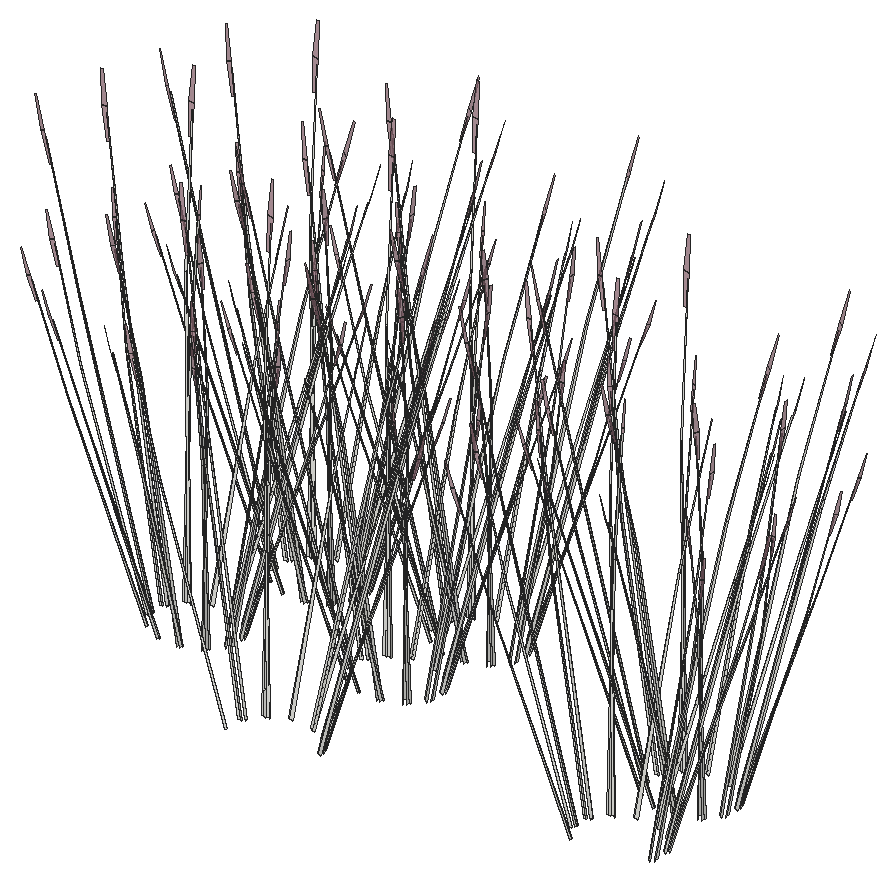
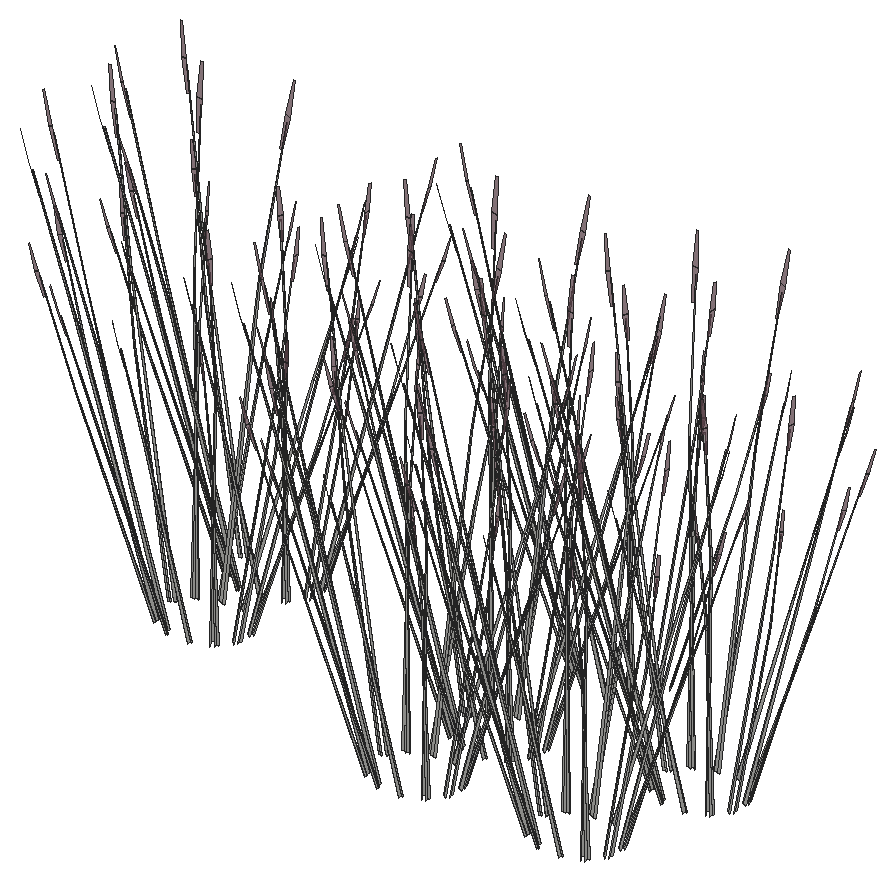
# SketchUp Ruby script. Lengths in inches.
U = 1.inch
M = Sketchup.active_model
def pt(a) = Geom::Point3d.new(a.map { |v| v * U })
def face(e, loops, mat)
  f = e.add_face(loops[0].map { |a| pt(a) })
  loops[1..].each { |l| e.add_face(l.map { |a| pt(a) }).erase! }
  f.material = f.back_material = mat if mat
  f
end
# faces: each face lists its corners as indices into pts; further lists are holes
def faces(e, pts, list, mat = nil) = list.each { |f| face(e, (f[0].is_a?(Array) ? f : [f]).map { |l| l.map { |i| pts[i] } }, mat) }
# xy, xz, yz: faces in a plane at the given z, y or x. An outline is a flat list of corners, or four numbers for a rectangle; further outlines are holes
def ring(l) = l.size == 4 ? [[l[0], l[1]], [l[2], l[1]], [l[2], l[3]], [l[0], l[3]]] : l.each_slice(2).to_a
def flat(e, list, mat, &to3) = list.each { |f| face(e, (f[0].is_a?(Array) ? f : [f]).map { |l| ring(l).map { |u, v| to3.(u, v) } }, mat) }
def xy(e, z, list, mat = nil) = flat(e, list, mat) { |x, y| [x, y, z] }
def xz(e, y, list, mat = nil) = flat(e, list, mat) { |x, z| [x, y, z] }
def yz(e, x, list, mat = nil) = flat(e, list, mat) { |y, z| [x, y, z] }
def lines(e, pts, list) = list.each { |a, b| e.add_line(pt(pts[a]), pt(pts[b])) }
# prism: a flat outline (further loops are holes) pulled along v
def prism(e, loops, v, mat = nil)
  f = face(e, loops, mat); d = Geom::Vector3d.new(v.map { |x| x * U })
  f.pushpull(f.normal.samedirection?(d) ? d.length : -d.length)
end
def box(e, o, s, mat = nil) = prism(e, [[o, [o[0] + s[0], o[1], o[2]], [o[0] + s[0], o[1] + s[1], o[2]], [o[0], o[1] + s[1], o[2]]]], [0, 0, s[2]], mat)
def at(x, y, z, deg = 0) = Geom::Transformation.translation(pt([x, y, z])) * Geom::Transformation.rotation(ORIGIN, Z_AXIS, deg.degrees)
def axes(o, x, y, z) = Geom::Transformation.new([*x, 0, *y, 0, *z, 0, *pt(o).to_a, 1])
def part(name) = M.definitions.add(name)
# library, detail: a bought-in or finely detailed component or shape, given as its bounding box
def library(name, o, s) = part(name).tap { |d| box(d.entities, o, s) }
def detail(e, o, s) = box(e.add_group.entities, o, s)
def put(e, d, t, mat = nil) = e.add_instance(d, t).tap { |i| i.material = mat if mat }
def group(e, t, mat = nil) = e.add_group.tap { |g| g.transformation = t; g.material = mat if mat }.entities
root = M.entities
M.materials.add("LightPink_Translucent").color = [144, 107, 117]
M.materials["LightPink_Translucent"].alpha = 0.75
c1 = part("blade")
p = [[2.15,0.21,22],[0,0.17,0],[0.09,0.45,0],[2.18,0.31,22],[2.29,0.31,22],[0.38,0.45,0],
  [2.48,0.24,33],[2.49,0.24,33],[2.48,0.22,33]]
faces(c1.entities,p,[[0,1,2,3],[4,5,2,3],[6,3,4,7],[8,0,3,6]])
c2 = part("seeds")
p = [[0.3,-0.1,1.38],[-0.01,-0.03,1.59],[-0.01,-0.03,0.03],[0.14,-0.07,-0.07],[0.29,-0.03,3],[0.15,0.01,3.11]]
faces(c2.entities,p,[[0,1,2,3],[1,0,4,5]],"LightPink_Translucent")
c3 = part("blade with seeds")
put(c3.entities,c1,at(0,0,0))
put(c3.entities,c2,axes([2.4,0.25,30.99],[1.5799,-0.05474,1.17369],[-0.12525,1.92788,0.29478],[-0.07173,-0.02425,1.56792]))
put(root,c3,axes([674.05,332.48,513.93],[-0.23895,-0.38931,0.05337],[0.43573,-0.19055,0.42015],[-0.19208,0.0376,0.64067]))
put(root,c3,axes([696.97,334.57,513.93],[0.03276,-0.43418,0.05337],[0.49468,0.0119,0.42015],[-0.18949,-0.04543,0.64067]))
put(root,c3,axes([680.24,333.61,513.93],[0.23895,0.38931,0.05337],[-0.43573,0.19055,0.42015],[0.19208,-0.0376,0.64067]))
put(root,c3,axes([680.2,333.47,513.93],[-0.18381,0.5206,0.39842],[-0.60429,-0.17802,0.32852],[0.23764,-0.03129,0.82444]))
put(root,c3,axes([702.34,335.55,513.93],[0.44663,0.24013,0.05337],[-0.26003,0.34195,0.42015],[0.14319,-0.11055,0.64067]))
put(root,c3,axes([702.21,335.45,513.93],[0.16135,0.52549,0.39842],[-0.63294,0.0912,0.32852],[0.18654,-0.12359,0.82444]))
put(root,c3,axes([666.05,338.03,513.93],[0.64106,0.14927,0.39842],[-0.21921,0.49074,0.32852],[-0.03852,-0.19299,0.82444]))
put(root,c3,axes([666.22,337.99,513.93],[0.47939,-0.19405,0.05337],[0.23464,0.35385,0.42015],[-0.0463,-0.15598,0.64067]))
put(root,c3,axes([674.24,333.91,513.93],[-0.16135,-0.52549,0.39842],[0.63294,-0.0912,0.32852],[-0.18654,0.12359,0.82444]))
put(root,c3,axes([674.11,333.81,513.93],[-0.44663,-0.24013,0.05337],[0.26003,-0.34195,0.42015],[-0.14319,0.11055,0.64067]))
put(root,c3,axes([664.57,338.04,513.93],[0.29569,-0.36271,0.05337],[0.42107,0.21117,0.42015],[-0.13613,-0.11629,0.64067]))
put(root,c3,axes([696.25,335.89,513.93],[0.18381,-0.5206,0.39842],[0.60429,0.17802,0.32852],[-0.23764,0.03129,0.82444]))
put(root,c3,axes([696.21,335.75,513.93],[-0.23895,-0.38931,0.05337],[0.43573,-0.19055,0.42015],[-0.19208,0.0376,0.64067]))
put(root,c3,axes([667.5,338.57,513.93],[0.46327,0.38957,0.39842],[-0.49199,0.33598,0.32852],[0.08546,-0.18277,0.82444]))
put(root,c3,axes([667.67,338.61,513.93],[0.53464,0.0266,0.05337],[-0.01466,0.40172,0.42015],[0.05594,-0.15388,0.64067]))
put(root,c3,axes([679.48,334.79,513.93],[-0.03276,0.43418,0.05337],[-0.49468,-0.0119,0.42015],[0.18949,0.04543,0.64067]))
put(root,c3,axes([679.53,334.65,513.93],[-0.47971,0.37622,0.39842],[-0.41372,-0.39954,0.32852],[0.22506,0.0694,0.82444]))
put(root,c3,axes([702.41,336.88,513.93],[0.23895,0.38931,0.05337],[-0.43573,0.19055,0.42015],[0.19208,-0.0376,0.64067]))
put(root,c3,axes([702.36,336.75,513.93],[-0.18381,0.5206,0.39842],[-0.60429,-0.17802,0.32852],[0.23764,-0.03129,0.82444]))
put(root,c3,axes([678.66,340.24,513.93],[0.64106,0.14927,0.39842],[-0.21921,0.49074,0.32852],[-0.03852,-0.19299,0.82444]))
put(root,c3,axes([699.83,340.24,513.93],[0.64106,0.14927,0.39842],[-0.21921,0.49074,0.32852],[-0.03852,-0.19299,0.82444]))
put(root,c3,axes([678.83,340.2,513.93],[0.47939,-0.19405,0.05337],[0.23464,0.35385,0.42015],[-0.0463,-0.15598,0.64067]))
put(root,c3,axes([700,340.2,513.93],[0.47939,-0.19405,0.05337],[0.23464,0.35385,0.42015],[-0.0463,-0.15598,0.64067]))
put(root,c3,axes([663.19,338.76,513.93],[0.03276,-0.43418,0.05337],[0.49468,0.0119,0.42015],[-0.18949,-0.04543,0.64067]))
put(root,c3,axes([674.99,334.9375,513.93],[-0.53464,-0.0266,0.05337],[0.01466,-0.40172,0.42015],[-0.05594,0.15388,0.64067]))
put(root,c3,axes([675.16,334.97,513.93],[-0.46327,-0.38957,0.39842],[0.49199,-0.33598,0.32852],[-0.08546,0.18277,0.82444]))
put(root,c3,axes([677.1875,340.26,513.93],[0.29569,-0.36271,0.05337],[0.42107,0.21117,0.42015],[-0.13613,-0.11629,0.64067]))
put(root,c3,axes([698.36,340.26,513.93],[0.29569,-0.36271,0.05337],[0.42107,0.21117,0.42015],[-0.13613,-0.11629,0.64067]))
put(root,c3,axes([678.09,335.5,513.93],[-0.29569,0.36271,0.05337],[-0.42107,-0.21117,0.42015],[0.13613,0.11629,0.64067]))
put(root,c3,axes([680.12,340.79,513.93],[0.46327,0.38957,0.39842],[-0.49199,0.33598,0.32852],[0.08546,-0.18277,0.82444]))
put(root,c3,axes([701.29,340.79,513.93],[0.46327,0.38957,0.39842],[-0.49199,0.33598,0.32852],[0.08546,-0.18277,0.82444]))
put(root,c3,axes([668.55,339.74,513.93],[0.44663,0.24013,0.05337],[-0.26003,0.34195,0.42015],[0.14319,-0.11055,0.64067]))
put(root,c3,axes([680.29,340.82,513.93],[0.53464,0.0266,0.05337],[-0.01466,0.40172,0.42015],[0.05594,-0.15388,0.64067]))
put(root,c3,axes([701.46,340.82,513.93],[0.53464,0.0266,0.05337],[-0.01466,0.40172,0.42015],[0.05594,-0.15388,0.64067]))
put(root,c3,axes([668.43,339.64,513.93],[0.16135,0.52549,0.39842],[-0.63294,0.0912,0.32852],[0.18654,-0.12359,0.82444]))
put(root,c3,axes([678.22,335.4,513.93],[-0.64708,0.13103,0.39842],[-0.1123,-0.514,0.32852],[0.15218,0.15149,0.82444]))
put(root,c3,axes([676.45,335.56,513.93],[-0.47939,0.19405,0.05337],[-0.23464,-0.35385,0.42015],[0.0463,0.15598,0.64067]))
put(root,c3,axes([696.4,337.1875,513.93],[-0.16135,-0.52549,0.39842],[0.63294,-0.0912,0.32852],[-0.18654,0.12359,0.82444]))
put(root,c3,axes([696.28,337.09,513.93],[-0.44663,-0.24013,0.05337],[0.26003,-0.34195,0.42015],[-0.14319,0.11055,0.64067]))
put(root,c3,axes([701.64,338.07,513.93],[-0.03276,0.43418,0.05337],[-0.49468,-0.0119,0.42015],[0.18949,0.04543,0.64067]))
put(root,c3,axes([675.8,340.97,513.93],[0.03276,-0.43418,0.05337],[0.49468,0.0119,0.42015],[-0.18949,-0.04543,0.64067]))
put(root,c3,axes([696.97,340.97,513.93],[0.03276,-0.43418,0.05337],[0.49468,0.0119,0.42015],[-0.18949,-0.04543,0.64067]))
put(root,c3,axes([701.6875,337.93,513.93],[-0.47971,0.37622,0.39842],[-0.41372,-0.39954,0.32852],[0.22506,0.0694,0.82444]))
put(root,c3,axes([662.47,340.08,513.93],[0.18381,-0.5206,0.39842],[0.60429,0.17802,0.32852],[-0.23764,0.03129,0.82444]))
put(root,c3,axes([662.42,339.94,513.93],[-0.23895,-0.38931,0.05337],[0.43573,-0.19055,0.42015],[-0.19208,0.0376,0.64067]))
put(root,c3,axes([681.17,341.95,513.93],[0.44663,0.24013,0.05337],[-0.26003,0.34195,0.42015],[0.14319,-0.11055,0.64067]))
put(root,c3,axes([702.34,341.95,513.93],[0.44663,0.24013,0.05337],[-0.26003,0.34195,0.42015],[0.14319,-0.11055,0.64067]))
put(root,c3,axes([681.04,341.85,513.93],[0.16135,0.52549,0.39842],[-0.63294,0.0912,0.32852],[0.18654,-0.12359,0.82444]))
put(root,c3,axes([702.21,341.85,513.93],[0.16135,0.52549,0.39842],[-0.63294,0.0912,0.32852],[0.18654,-0.12359,0.82444]))
put(root,c3,axes([697.15,338.21,513.93],[-0.53464,-0.0266,0.05337],[0.01466,-0.40172,0.42015],[-0.05594,0.15388,0.64067]))
put(root,c3,axes([697.32,338.25,513.93],[-0.46327,-0.38957,0.39842],[0.49199,-0.33598,0.32852],[-0.08546,0.18277,0.82444]))
put(root,c3,axes([668.62,341.07,513.93],[0.23895,0.38931,0.05337],[-0.43573,0.19055,0.42015],[0.19208,-0.0376,0.64067]))
put(root,c3,axes([668.57,340.93,513.93],[-0.18381,0.5206,0.39842],[-0.60429,-0.17802,0.32852],[0.23764,-0.03129,0.82444]))
put(root,c3,axes([700.25,338.78,513.93],[-0.29569,0.36271,0.05337],[-0.42107,-0.21117,0.42015],[0.13613,0.11629,0.64067]))
put(root,c3,axes([700.375,338.68,513.93],[-0.64708,0.13103,0.39842],[-0.1123,-0.514,0.32852],[0.15218,0.15149,0.82444]))
put(root,c3,axes([698.61,338.83,513.93],[-0.47939,0.19405,0.05337],[-0.23464,-0.35385,0.42015],[0.0463,0.15598,0.64067]))
put(root,c3,axes([675.08,342.29,513.93],[0.18381,-0.5206,0.39842],[0.60429,0.17802,0.32852],[-0.23764,0.03129,0.82444]))
put(root,c3,axes([696.25,342.29,513.93],[0.18381,-0.5206,0.39842],[0.60429,0.17802,0.32852],[-0.23764,0.03129,0.82444]))
put(root,c3,axes([675.04,342.15,513.93],[-0.23895,-0.38931,0.05337],[0.43573,-0.19055,0.42015],[-0.19208,0.0376,0.64067]))
put(root,c3,axes([696.21,342.15,513.93],[-0.23895,-0.38931,0.05337],[0.43573,-0.19055,0.42015],[-0.19208,0.0376,0.64067]))
put(root,c3,axes([662.61,341.375,513.93],[-0.16135,-0.52549,0.39842],[0.63294,-0.0912,0.32852],[-0.18654,0.12359,0.82444]))
put(root,c3,axes([662.49,341.27,513.93],[-0.44663,-0.24013,0.05337],[0.26003,-0.34195,0.42015],[-0.14319,0.11055,0.64067]))
put(root,c3,axes([668.3,346.37,513.93],[0.64106,0.14927,0.39842],[-0.21921,0.49074,0.32852],[-0.03852,-0.19299,0.82444]))
put(root,c3,axes([681.23,343.28,513.93],[0.23895,0.38931,0.05337],[-0.43573,0.19055,0.42015],[0.19208,-0.0376,0.64067]))
put(root,c3,axes([702.41,343.28,513.93],[0.23895,0.38931,0.05337],[-0.43573,0.19055,0.42015],[0.19208,-0.0376,0.64067]))
put(root,c3,axes([681.1875,343.15,513.93],[-0.18381,0.5206,0.39842],[-0.60429,-0.17802,0.32852],[0.23764,-0.03129,0.82444]))
put(root,c3,axes([702.36,343.15,513.93],[-0.18381,0.5206,0.39842],[-0.60429,-0.17802,0.32852],[0.23764,-0.03129,0.82444]))
put(root,c3,axes([668.47,346.33,513.93],[0.47939,-0.19405,0.05337],[0.23464,0.35385,0.42015],[-0.0463,-0.15598,0.64067]))
put(root,c3,axes([679.61,346.57,513.93],[0.64106,0.14927,0.39842],[-0.21921,0.49074,0.32852],[-0.03852,-0.19299,0.82444]))
put(root,c3,axes([679.78,346.53,513.93],[0.47939,-0.19405,0.05337],[0.23464,0.35385,0.42015],[-0.0463,-0.15598,0.64067]))
put(root,c3,axes([667.85,342.25,513.93],[-0.03276,0.43418,0.05337],[-0.49468,-0.0119,0.42015],[0.18949,0.04543,0.64067]))
put(root,c3,axes([666.83,346.39,513.93],[0.29569,-0.36271,0.05337],[0.42107,0.21117,0.42015],[-0.13613,-0.11629,0.64067]))
put(root,c3,axes([667.9,342.12,513.93],[-0.47971,0.37622,0.39842],[-0.41372,-0.39954,0.32852],[0.22506,0.0694,0.82444]))
put(root,c3,axes([678.14,346.59,513.93],[0.29569,-0.36271,0.05337],[0.42107,0.21117,0.42015],[-0.13613,-0.11629,0.64067]))
put(root,c3,axes([669.76,346.91,513.93],[0.46327,0.38957,0.39842],[-0.49199,0.33598,0.32852],[0.08546,-0.18277,0.82444]))
put(root,c3,axes([669.93,346.95,513.93],[0.53464,0.0266,0.05337],[-0.01466,0.40172,0.42015],[0.05594,-0.15388,0.64067]))
put(root,c3,axes([681.07,347.12,513.93],[0.46327,0.38957,0.39842],[-0.49199,0.33598,0.32852],[0.08546,-0.18277,0.82444]))
put(root,c3,axes([681.24,347.15,513.93],[0.53464,0.0266,0.05337],[-0.01466,0.40172,0.42015],[0.05594,-0.15388,0.64067]))
put(root,c3,axes([675.23,343.59,513.93],[-0.16135,-0.52549,0.39842],[0.63294,-0.0912,0.32852],[-0.18654,0.12359,0.82444]))
put(root,c3,axes([696.4,343.59,513.93],[-0.16135,-0.52549,0.39842],[0.63294,-0.0912,0.32852],[-0.18654,0.12359,0.82444]))
put(root,c3,axes([663.37,342.4,513.93],[-0.53464,-0.0266,0.05337],[0.01466,-0.40172,0.42015],[-0.05594,0.15388,0.64067]))
put(root,c3,axes([675.1,343.49,513.93],[-0.44663,-0.24013,0.05337],[0.26003,-0.34195,0.42015],[-0.14319,0.11055,0.64067]))
put(root,c3,axes([696.28,343.49,513.93],[-0.44663,-0.24013,0.05337],[0.26003,-0.34195,0.42015],[-0.14319,0.11055,0.64067]))
put(root,c3,axes([663.54,342.4375,513.93],[-0.46327,-0.38957,0.39842],[0.49199,-0.33598,0.32852],[-0.08546,0.18277,0.82444]))
put(root,c3,axes([666.47,342.97,513.93],[-0.29569,0.36271,0.05337],[-0.42107,-0.21117,0.42015],[0.13613,0.11629,0.64067]))
put(root,c3,axes([665.44,347.1,513.93],[0.03276,-0.43418,0.05337],[0.49468,0.0119,0.42015],[-0.18949,-0.04543,0.64067]))
put(root,c3,axes([666.59,342.87,513.93],[-0.64708,0.13103,0.39842],[-0.1123,-0.514,0.32852],[0.15218,0.15149,0.82444]))
put(root,c3,axes([676.75,347.3,513.93],[0.03276,-0.43418,0.05337],[0.49468,0.0119,0.42015],[-0.18949,-0.04543,0.64067]))
put(root,c3,axes([680.47,344.47,513.93],[-0.03276,0.43418,0.05337],[-0.49468,-0.0119,0.42015],[0.18949,0.04543,0.64067]))
put(root,c3,axes([701.64,344.47,513.93],[-0.03276,0.43418,0.05337],[-0.49468,-0.0119,0.42015],[0.18949,0.04543,0.64067]))
put(root,c3,axes([680.51,344.33,513.93],[-0.47971,0.37622,0.39842],[-0.41372,-0.39954,0.32852],[0.22506,0.0694,0.82444]))
put(root,c3,axes([701.6875,344.33,513.93],[-0.47971,0.37622,0.39842],[-0.41372,-0.39954,0.32852],[0.22506,0.0694,0.82444]))
put(root,c3,axes([664.82,343.02,513.93],[-0.47939,0.19405,0.05337],[-0.23464,-0.35385,0.42015],[0.0463,0.15598,0.64067]))
put(root,c3,axes([670.81,348.08,513.93],[0.44663,0.24013,0.05337],[-0.26003,0.34195,0.42015],[0.14319,-0.11055,0.64067]))
put(root,c3,axes([670.68,347.98,513.93],[0.16135,0.52549,0.39842],[-0.63294,0.0912,0.32852],[0.18654,-0.12359,0.82444]))
put(root,c3,axes([682.12,348.28,513.93],[0.44663,0.24013,0.05337],[-0.26003,0.34195,0.42015],[0.14319,-0.11055,0.64067]))
put(root,c3,axes([681.99,348.18,513.93],[0.16135,0.52549,0.39842],[-0.63294,0.0912,0.32852],[0.18654,-0.12359,0.82444]))
put(root,c3,axes([675.98,344.61,513.93],[-0.53464,-0.0266,0.05337],[0.01466,-0.40172,0.42015],[-0.05594,0.15388,0.64067]))
put(root,c3,axes([697.15,344.61,513.93],[-0.53464,-0.0266,0.05337],[0.01466,-0.40172,0.42015],[-0.05594,0.15388,0.64067]))
put(root,c3,axes([676.15,344.65,513.93],[-0.46327,-0.38957,0.39842],[0.49199,-0.33598,0.32852],[-0.08546,0.18277,0.82444]))
put(root,c3,axes([697.32,344.65,513.93],[-0.46327,-0.38957,0.39842],[0.49199,-0.33598,0.32852],[-0.08546,0.18277,0.82444]))
put(root,c3,axes([679.08,345.18,513.93],[-0.29569,0.36271,0.05337],[-0.42107,-0.21117,0.42015],[0.13613,0.11629,0.64067]))
put(root,c3,axes([700.25,345.18,513.93],[-0.29569,0.36271,0.05337],[-0.42107,-0.21117,0.42015],[0.13613,0.11629,0.64067]))
put(root,c3,axes([679.2,345.08,513.93],[-0.64708,0.13103,0.39842],[-0.1123,-0.514,0.32852],[0.15218,0.15149,0.82444]))
put(root,c3,axes([700.375,345.08,513.93],[-0.64708,0.13103,0.39842],[-0.1123,-0.514,0.32852],[0.15218,0.15149,0.82444]))
put(root,c3,axes([677.4375,345.23,513.93],[-0.47939,0.19405,0.05337],[-0.23464,-0.35385,0.42015],[0.0463,0.15598,0.64067]))
put(root,c3,axes([698.61,345.23,513.93],[-0.47939,0.19405,0.05337],[-0.23464,-0.35385,0.42015],[0.0463,0.15598,0.64067]))
put(root,c3,axes([664.73,348.42,513.93],[0.18381,-0.5206,0.39842],[0.60429,0.17802,0.32852],[-0.23764,0.03129,0.82444]))
put(root,c3,axes([664.68,348.28,513.93],[-0.23895,-0.38931,0.05337],[0.43573,-0.19055,0.42015],[-0.19208,0.0376,0.64067]))
put(root,c3,axes([676.03,348.62,513.93],[0.18381,-0.5206,0.39842],[0.60429,0.17802,0.32852],[-0.23764,0.03129,0.82444]))
put(root,c3,axes([675.99,348.48,513.93],[-0.23895,-0.38931,0.05337],[0.43573,-0.19055,0.42015],[-0.19208,0.0376,0.64067]))
put(root,c3,axes([670.875,349.41,513.93],[0.23895,0.38931,0.05337],[-0.43573,0.19055,0.42015],[0.19208,-0.0376,0.64067]))
put(root,c3,axes([670.83,349.27,513.93],[-0.18381,0.5206,0.39842],[-0.60429,-0.17802,0.32852],[0.23764,-0.03129,0.82444]))
put(root,c3,axes([682.18,349.62,513.93],[0.23895,0.38931,0.05337],[-0.43573,0.19055,0.42015],[0.19208,-0.0376,0.64067]))
put(root,c3,axes([682.14,349.48,513.93],[-0.18381,0.5206,0.39842],[-0.60429,-0.17802,0.32852],[0.23764,-0.03129,0.82444]))
put(root,c3,axes([664.87,349.72,513.93],[-0.16135,-0.52549,0.39842],[0.63294,-0.0912,0.32852],[-0.18654,0.12359,0.82444]))
put(root,c3,axes([664.75,349.62,513.93],[-0.44663,-0.24013,0.05337],[0.26003,-0.34195,0.42015],[-0.14319,0.11055,0.64067]))
put(root,c3,axes([676.18,349.92,513.93],[-0.16135,-0.52549,0.39842],[0.63294,-0.0912,0.32852],[-0.18654,0.12359,0.82444]))
put(root,c3,axes([676.05,349.82,513.93],[-0.44663,-0.24013,0.05337],[0.26003,-0.34195,0.42015],[-0.14319,0.11055,0.64067]))
put(root,c3,axes([670.11,350.6,513.93],[-0.03276,0.43418,0.05337],[-0.49468,-0.0119,0.42015],[0.18949,0.04543,0.64067]))
put(root,c3,axes([670.16,350.46,513.93],[-0.47971,0.37622,0.39842],[-0.41372,-0.39954,0.32852],[0.22506,0.0694,0.82444]))
put(root,c3,axes([681.42,350.8,513.93],[-0.03276,0.43418,0.05337],[-0.49468,-0.0119,0.42015],[0.18949,0.04543,0.64067]))
put(root,c3,axes([681.47,350.66,513.93],[-0.47971,0.37622,0.39842],[-0.41372,-0.39954,0.32852],[0.22506,0.0694,0.82444]))
put(root,c3,axes([665.625,350.74,513.93],[-0.53464,-0.0266,0.05337],[0.01466,-0.40172,0.42015],[-0.05594,0.15388,0.64067]))
put(root,c3,axes([665.8,350.78,513.93],[-0.46327,-0.38957,0.39842],[0.49199,-0.33598,0.32852],[-0.08546,0.18277,0.82444]))
put(root,c3,axes([676.93,350.95,513.93],[-0.53464,-0.0266,0.05337],[0.01466,-0.40172,0.42015],[-0.05594,0.15388,0.64067]))
put(root,c3,axes([677.1,350.98,513.93],[-0.46327,-0.38957,0.39842],[0.49199,-0.33598,0.32852],[-0.08546,0.18277,0.82444]))
put(root,c3,axes([668.72,351.31,513.93],[-0.29569,0.36271,0.05337],[-0.42107,-0.21117,0.42015],[0.13613,0.11629,0.64067]))
put(root,c3,axes([668.85,351.21,513.93],[-0.64708,0.13103,0.39842],[-0.1123,-0.514,0.32852],[0.15218,0.15149,0.82444]))
put(root,c3,axes([680.03,351.51,513.93],[-0.29569,0.36271,0.05337],[-0.42107,-0.21117,0.42015],[0.13613,0.11629,0.64067]))
put(root,c3,axes([680.16,351.41,513.93],[-0.64708,0.13103,0.39842],[-0.1123,-0.514,0.32852],[0.15218,0.15149,0.82444]))
put(root,c3,axes([667.08,351.36,513.93],[-0.47939,0.19405,0.05337],[-0.23464,-0.35385,0.42015],[0.0463,0.15598,0.64067]))
put(root,c3,axes([678.39,351.57,513.93],[-0.47939,0.19405,0.05337],[-0.23464,-0.35385,0.42015],[0.0463,0.15598,0.64067]))
